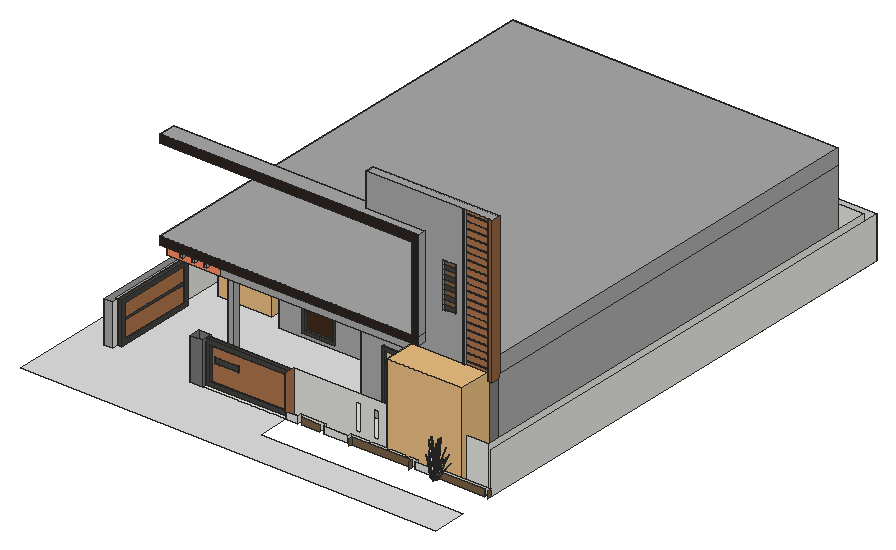
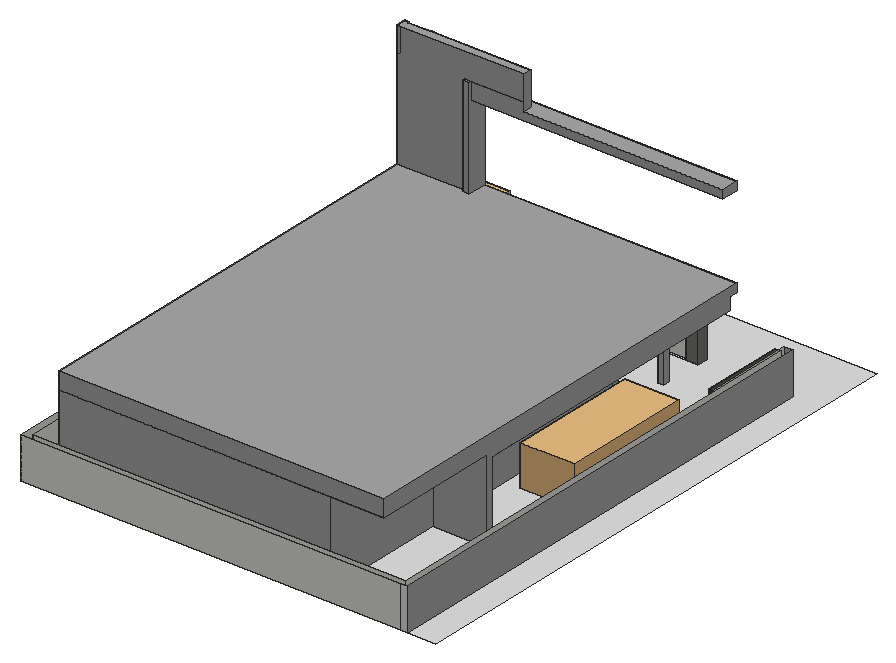
# SketchUp Ruby script. Lengths in inches.
U = 1.inch
M = Sketchup.active_model
def pt(a) = Geom::Point3d.new(a.map { |v| v * U })
def face(e, loops, mat)
  f = e.add_face(loops[0].map { |a| pt(a) })
  loops[1..].each { |l| e.add_face(l.map { |a| pt(a) }).erase! }
  f.material = f.back_material = mat if mat
  f
end
# faces: each face lists its corners as indices into pts; further lists are holes
def faces(e, pts, list, mat = nil) = list.each { |f| face(e, (f[0].is_a?(Array) ? f : [f]).map { |l| l.map { |i| pts[i] } }, mat) }
# xy, xz, yz: faces in a plane at the given z, y or x. An outline is a flat list of corners, or four numbers for a rectangle; further outlines are holes
def ring(l) = l.size == 4 ? [[l[0], l[1]], [l[2], l[1]], [l[2], l[3]], [l[0], l[3]]] : l.each_slice(2).to_a
def flat(e, list, mat, &to3) = list.each { |f| face(e, (f[0].is_a?(Array) ? f : [f]).map { |l| ring(l).map { |u, v| to3.(u, v) } }, mat) }
def xy(e, z, list, mat = nil) = flat(e, list, mat) { |x, y| [x, y, z] }
def xz(e, y, list, mat = nil) = flat(e, list, mat) { |x, z| [x, y, z] }
def yz(e, x, list, mat = nil) = flat(e, list, mat) { |y, z| [x, y, z] }
def lines(e, pts, list) = list.each { |a, b| e.add_line(pt(pts[a]), pt(pts[b])) }
# prism: a flat outline (further loops are holes) pulled along v
def prism(e, loops, v, mat = nil)
  f = face(e, loops, mat); d = Geom::Vector3d.new(v.map { |x| x * U })
  f.pushpull(f.normal.samedirection?(d) ? d.length : -d.length)
end
def box(e, o, s, mat = nil) = prism(e, [[o, [o[0] + s[0], o[1], o[2]], [o[0] + s[0], o[1] + s[1], o[2]], [o[0], o[1] + s[1], o[2]]]], [0, 0, s[2]], mat)
def at(x, y, z, deg = 0) = Geom::Transformation.translation(pt([x, y, z])) * Geom::Transformation.rotation(ORIGIN, Z_AXIS, deg.degrees)
def axes(o, x, y, z) = Geom::Transformation.new([*x, 0, *y, 0, *z, 0, *pt(o).to_a, 1])
def part(name) = M.definitions.add(name)
# library, detail: a bought-in or finely detailed component or shape, given as its bounding box
def library(name, o, s) = part(name).tap { |d| box(d.entities, o, s) }
def detail(e, o, s) = box(e.add_group.entities, o, s)
def put(e, d, t, mat = nil) = e.add_instance(d, t).tap { |i| i.material = mat if mat }
def group(e, t, mat = nil) = e.add_group.tap { |g| g.transformation = t; g.material = mat if mat }.entities
root = M.entities
M.materials.add("B03_Apricot_Glow").color = [255, 140, 101]
M.materials.add("Glass_Mirror_01").color = [226, 201, 168]
M.materials["Glass_Mirror_01"].alpha = 0.74
M.materials.add("Image").color = [118, 118, 115]
M.materials.add("M01_Silver_Fog").color = [224, 224, 224]
M.materials.add("M03_Pewter_Shine").color = [168, 168, 168]
M.materials.add("Plywood_01_1K").color = [125, 96, 64]
M.materials.add("Soil_03_1K").color = [122, 96, 67]
M.materials.add("Wood_Floor_12_1K").color = [45, 37, 32]
M.materials.add("Wood_Planks_01_1K").color = [69, 67, 63]
M.materials.add("Wood_Veneer_15_1K").color = [173, 116, 75]
M.materials.add("Wood_Veneer_15_1K1").color = [147, 99, 64]
M.materials.add("Wood_Veneer_15_1K2").color = [173, 116, 75]
M.materials.add("Wood_Veneer_15_1K3").color = [66, 44, 28]
c1 = part("blade")
p = [[2.15,0.21,22],[0,0.17,0],[0.09,0.45,0],[2.18,0.31,22],[2.29,0.31,22],[0.38,0.45,0],
  [2.48,0.24,33],[2.49,0.24,33],[2.48,0.22,33]]
faces(c1.entities,p,[[0,1,2,3],[4,5,2,3],[6,3,4,7],[8,0,3,6]])
c2 = part("blade with seeds\#1")
put(c2.entities,c1,at(0,0,0))
c3 = library("Baneira",[-21.22,-27.99,0],[51.24,48.13,67.625])
c4 = library("Car Sedan",[0,-0.48,0],[188.37,78.26,58.82])
xy(root,0,[[307.48,94.87,325.48,94.87,325.48,100.87,361.48,100.87,361.48,95.87,397.48,95.87,397.48,100.87,493.75,100.87,493.75,95.87,517.75,95.87,517.75,100.87,600,100.87,600,796.87,49.48,796.87,49.48,788.61,588.83,788.61,588.83,109.87,307.48,109.87],[169.48,94.87,187.48,109.87],[187.48,94.87,307.48,100.87],[187.48,100.87,307.48,109.87]])
xy(root,0,[[0,0,600.39,0,600.39,49.75,307.48,49.75,307.48,94.87,169.48,94.87,169.48,109.87,588.83,109.87,588.83,788.61,49.48,788.61,49.48,109.87,52.41,109.87,52.41,100.87,40.48,100.87,40.48,796.87,0,796.87]],"M01_Silver_Fog")
xz(root,94.87,[[307.48,0,325.48,10]])
xz(root,94.87,[[169.48,0,187.48,60]],"Image")
xz(root,95.87,[[361.48,0,397.48,10],[493.75,0,517.75,10]])
xz(root,95.87,[[330.48,0,356.48,10],[402.48,0,488.75,10],[522.75,0,595,10]],"Soil_03_1K")
xz(root,100.87,[[325.48,0,361.48,10],[397.48,0,493.75,0,493.75,10,482.46,10,482.46,9.35,475.45,9.35,475.45,10,456.47,10,456.47,9.35,449.46,9.35,449.46,10,430.48,10,430.48,9.35,423.47,9.35,423.47,10,404.48,10,404.48,9.35,397.48,9.35],[517.75,0,600,10]])
xz(root,100.87,[[40.48,0,52.41,60]],"M03_Pewter_Shine")
xz(root,109.87,[[49.48,0,52.41,60],[[307.48,0,588.83,60],[475.45,9.35,482.46,48],[449.46,9.35,456.47,48],[423.47,9.35,430.48,48],[397.48,9.35,404.48,48]]])
xz(root,109.87,[[169.48,0,187.48,60]],"Image")
xz(root,788.61,[[49.48,0,588.83,60]])
xz(root,796.87,[[40.48,0,49.48,60],[49.48,0,600,60]])
yz(root,40.48,[[100.87,0,796.87,60]],"M03_Pewter_Shine")
yz(root,49.48,[[109.87,0,788.61,60]])
yz(root,52.41,[[100.87,0,109.87,60]])
yz(root,169.48,[[94.87,0,109.87,60]],"Image")
yz(root,187.48,[[94.87,0,109.87,60]],"Image")
yz(root,307.48,[[94.87,0,109.87,60]],"Wood_Veneer_15_1K2")
yz(root,325.48,[[94.87,0,100.87,10]])
yz(root,361.48,[[95.87,0,100.87,10]])
yz(root,397.48,[[95.87,0,100.87,10]])
yz(root,402.48,[[90.87,0,95.87,10]],"Soil_03_1K")
yz(root,488.75,[[90.87,0,95.87,10]],"Soil_03_1K")
yz(root,493.75,[[95.87,0,100.87,10]])
yz(root,517.75,[[95.87,0,100.87,10]])
yz(root,522.75,[[90.87,0,95.87,10]],"Soil_03_1K")
yz(root,588.83,[[109.87,0,788.61,60]])
yz(root,595,[[94.87,0,95.87,10]],"Soil_03_1K")
yz(root,600,[[100.87,0,796.87,60]])
yz(root,600,[[94.87,0,100.87,10]],"Soil_03_1K")
put(root,c2,axes([527.79,90.97,3.51],[0.90375,0.03008,-0.71091],[-0.0607,1.26677,0.08579],[0.38287,0.13368,1.00565]))
put(root,c2,axes([526.65,87.39,1.69],[0.39398,-0.99907,1.36359],[0.84877,0.97875,0.53923],[-0.50305,0.4384,1.14314]))
put(root,c2,axes([519.51,91.2,1.1875],[0.34005,-0.60308,1.03545],[0.20441,0.87829,0.76078],[-0.26134,0.18792,0.22807]))
put(root,c2,axes([526.79,87.49,0.55],[0.73437,0.77871,-0.5621],[-0.66591,0.96736,-0.14753],[0.18319,0.31204,1.24074]))
put(root,c2,axes([524.38,91.8125,0.8],[0.82143,1.07538,0.27726],[-0.81279,1.07603,-0.32897],[-0.23327,0.03755,1.48641]))
put(root,c2,axes([527.44,90.9,0.52],[-0.85134,0.27158,-0.27926],[-0.24175,-1.0786,0.27926],[-0.09817,0.21744,1.25283]))
put(root,c2,axes([520.68,90.09,2.78],[-0.78697,0.17856,-0.31925],[-0.2078,-1.02074,0.41216],[-0.22552,0.27417,0.78863]))
put(root,c2,axes([528.33,91.49,2.78],[0.51441,0.78225,-0.31925],[-0.58738,0.7405,0.41216],[0.29843,0.11267,0.78863]))
put(root,c2,axes([526.08,88.26,1.1],[0.64866,1.16728,-0.26229],[-0.91655,0.77622,-0.45076],[-0.09308,0.288,1.43974]))
put(root,c2,axes([524.67,92.93,0.83],[0,1.44565,0],[-1.09198,0,-0.46523],[-0.24871,0,1.47583]))
put(root,c2,axes([520.02,90.85,1.03],[0.31962,0.07001,1.28914],[0.26756,1.02347,-0.27724],[-0.41311,0.23924,0.55117]))
put(root,c2,axes([529.81,91.86,1.03],[-0.15413,-0.36483,1.28914],[0.46474,-0.90077,-0.27724],[0.40213,0.2681,0.55117]))
put(root,c2,axes([521.03,92.38,0.61],[0.7978,0.33351,-0.03509],[-0.24541,1.02647,-0.15911],[-0.13049,0.15585,0.52479]))
put(root,c2,axes([528.4,90.54,0.83],[0.97904,0.72283,0],[-0.54599,1.20931,-0.46523],[-0.12435,0.27543,1.47583]))
put(root,c2,axes([527.81,91.2,0.51],[-0.48852,1.08202,-0.44759],[-0.87598,-0.64674,0],[-0.11126,0.24644,1.41987]))
put(root,c2,axes([521.31,89.75,3.1875],[-0.47225,0.98582,-0.64046],[-0.82754,-0.7006,0.07729],[-0.28197,0.35717,0.906]))
put(root,c2,axes([520.53,91.68,0.04],[0.12871,0.11199,1.5897],[0.2775,1.13173,-0.24285],[-0.25244,0.2734,0.27078]))
put(root,c2,axes([521.33,90.21,2.92],[0.23225,1.14083,-0.46065],[-0.87956,0.19957,-0.35681],[-0.25205,0.30642,0.88141]))
put(root,c2,axes([525.9375,89.625,0.55],[-0.16018,1.20264,-0.5621],[-0.98808,-0.25378,-0.14753],[-0.11973,0.3589,1.24074]))
put(root,c2,axes([526.58,92.43,2.92],[0.89213,-0.297,-0.46065],[0.15606,1.12475,-0.35681],[0.23962,0.32232,0.88141]))
put(root,c2,axes([528.85,93.81,0.04],[0.09761,-0.15508,1.5897],[0.90442,-0.26295,-0.24285],[0.19286,0.3437,0.27078]))
put(root,c2,axes([523.53,94.03,1.1875],[-0.06991,-0.73811,1.03545],[0.616,0.4682,0.76078],[-0.09241,0.36475,0.22807]))
put(root,c2,axes([526.48,93.26,2.78],[0.13963,1.00636,-0.31925],[-0.79822,0.26574,0.41216],[0.2144,0.28839,0.78863]))
put(root,c2,axes([528.4,95.08,1.1875],[-0.44281,-0.48182,1.03545],[0.70101,-0.19012,0.76078],[0.12552,0.34819,0.22807]))
put(root,c2,axes([522.68,92.14,2.92],[0.6472,0.83949,-0.46065],[-0.68369,0.73521,-0.35681],[-0.09847,0.42653,0.88141]))
put(root,c2,axes([524.54,93.49,0.04],[0.15398,-0.02932,1.5897],[0.80412,0.59108,-0.24285],[-0.04053,0.41985,0.27078]))
put(root,c2,axes([524.6,92.95,2.92],[0.88873,0.31321,-0.46065],[-0.30463,1.07385,-0.35681],[0.08149,0.43235,0.88141]))
put(root,c2,axes([524.19,93.61,2.78],[-0.27256,0.96081,-0.31925],[-0.79518,-0.28024,0.41216],[0.07291,0.38684,0.78863]))
put(root,c2,axes([522.48,91.76,3.1875],[-0.02352,1.1557,-0.64046],[-0.99061,-0.07762,0.07729],[-0.10454,0.48961,0.906]))
put(root,c2,axes([522.72,92.6875,1.03],[0.27202,-0.22572,1.28914],[0.7394,0.52014,-0.27724],[-0.17673,0.53408,0.55117]))
put(root,c2,axes([524.06,90.69,1.71],[-0.14134,-0.32863,1.5962],[0.98684,-0.11332,0.12492],[0.13095,0.71181,0.57049]))
put(root,c2,axes([526.68,94.24,1.03],[0.08021,-0.40179,1.28914],[0.81924,-0.25896,-0.27724],[0.15335,0.54576,0.55117]))
g1 = group(root,at(187.48,106.87,0))
xy(g1,0,[[0,-6,120,0]],"Wood_Planks_01_1K")
xy(g1,6,[[6,-6,114,-3]],"Wood_Planks_01_1K")
xy(g1,29.67,[[10.07,-3,45.08,-1.64]],"Wood_Planks_01_1K")
xy(g1,38.71,[[10.07,-3,45.08,-1.64]],"Wood_Planks_01_1K")
xy(g1,54,[[6,-6,114,-3]],"Wood_Planks_01_1K")
xy(g1,60,[[0,-6,120,0]],"Wood_Planks_01_1K")
xz(g1,-6,[[[0,0,120,60],[6,6,114,54]]],"Wood_Planks_01_1K")
xz(g1,-3,[[[6,6,114,54],[10.07,29.67,45.08,38.71]]],"Wood_Veneer_15_1K2")
xz(g1,-1.64,[[10.07,29.67,45.08,38.71]],"Wood_Planks_01_1K")
xz(g1,0,[[0,0,120,60]])
yz(g1,0,[[-6,0,0,60]],"Wood_Planks_01_1K")
yz(g1,6,[[-6,6,-3,54]],"Wood_Planks_01_1K")
yz(g1,10.07,[[-3,29.67,-1.64,38.71]],"Wood_Planks_01_1K")
yz(g1,45.08,[[-3,29.67,-1.64,38.71]],"Wood_Planks_01_1K")
yz(g1,114,[[-6,6,-3,54]],"Wood_Planks_01_1K")
yz(g1,120,[[-6,0,0,60]],"Wood_Planks_01_1K")
put(root,c3,axes([492.54,131.13,0],[2.1112,0,0],[0,1,0],[0,0,1.8357]))
g2 = group(root,at(52.41,109.87,0,90))
xy(g2,0,[[0,-6,120,0]],"Wood_Planks_01_1K")
xy(g2,6,[[6,-6,114,-3]],"Wood_Planks_01_1K")
xy(g2,54,[[6,-6,114,-3]],"Wood_Planks_01_1K")
xy(g2,60,[[0,-6,120,0]],"Wood_Planks_01_1K")
xz(g2,-6,[[[0,0,120,60],[6,6,114,54]]],"Wood_Planks_01_1K")
xz(g2,-3,[[6,28,114,32]],"Wood_Planks_01_1K")
xz(g2,-3,[[6,6,114,28],[6,32,114,54]],"Wood_Veneer_15_1K2")
xz(g2,0,[[0,0,120,60]])
yz(g2,0,[[-6,0,0,60]],"Wood_Planks_01_1K")
yz(g2,6,[[-6,6,-3,54]],"Wood_Planks_01_1K")
yz(g2,114,[[-6,6,-3,54]],"Wood_Planks_01_1K")
yz(g2,120,[[-6,0,0,60]],"Wood_Planks_01_1K")
put(root,c4,at(148.51,268.88,0,90))
g3 = group(root,at(129,160.87,120),"M03_Pewter_Shine")
xy(g3,-120,[[-36,418.1,50.06,427.58]])
xy(g3,-6,[[393.23,-13.66,393.23,-12.74,40.22,-12.74,40.22,0,435,0,435,-13.66,429,-13.66,429,-12,395.99,-12,395.99,-13.66],[-36,-12.74,-36,418.1,-24.58,418.1,-24.58,0,40.22,0,40.22,-12.74]])
xy(g3,0,[[-24.58,0,-24.58,418.1,50.06,418.1,50.06,427.58,-36,427.58,-36,612,435,612,435,0]])
xy(g3,0.01,[[-14.8125,-16,-10.09,-12.74],[2.7,-16,7.42,-12.74],[20.21,-16,24.93,-12.74]])
xy(g3,4.51,[[-14.8125,-16,-10.09,-12.74],[2.7,-16,7.42,-12.74],[20.21,-16,24.93,-12.74]])
xy(g3,12,[[-36,-24.39,337.47,-12.74]])
xy(g3,24,[[-36,-24.39,328.3125,-24.39,328.3125,3.12,337.47,3.12,337.47,0,435,0,435,612,-36,612]])
xy(g3,63.78,[[363.53,-12.74,381.62,-12]])
xy(g3,128.54,[[363.53,-12.74,381.62,-12]])
xy(g3,144,[[-36,-24.39,328.3125,0]],"Wood_Floor_12_1K")
xy(g3,156,[[-36,-24.39,337.47,-24.39,337.47,-12.74,252.48,-12.74,252.48,0,-36,0]])
xy(g3,168,[[328.3125,0,337.47,3.12]])
xy(g3,204,[[393.23,-13.66,395.99,-13.66,395.99,-12,429,-12,429,-13.66,435,-13.66,435,0,252.48,0,252.48,-12.74,393.23,-12.74]])
xz(g3,-24.39,[[-36,12,337.47,12,337.47,156,-36,156,-36,144,328.3125,144,328.3125,24,-36,24]],"Wood_Floor_12_1K")
xz(g3,-16,[[-14.8125,0.01,-10.09,4.51],[2.7,0.01,7.42,4.51],[20.21,0.01,24.93,4.51]])
xz(g3,-13.66,[[393.23,-6,395.99,204]])
xz(g3,-13.66,[[429,-6,435,204]],"Wood_Veneer_15_1K1")
xz(g3,-12.74,[[[40.22,-6,393.23,-6,393.23,204,252.48,204,252.48,156,337.47,156,337.47,12,39.74,12],[363.53,63.78,381.62,128.54]]])
xz(g3,-12.74,[[[-36,-6,40.22,-6,39.74,12,-36,12],[-14.8125,0.01,-10.09,4.51],[2.7,0.01,7.42,4.51],[20.21,0.01,24.93,4.51]]],"B03_Apricot_Glow")
xz(g3,-12,[[395.99,-1.84,429,-0.84],[395.99,8.2,429,9.2],[395.99,18.25,429,19.25],[395.99,28.29,429,29.29],[395.99,38.33,429,39.33],
  [395.99,48.37,429,49.37],[395.99,58.41,429,59.41],[395.99,68.46,429,69.46],[395.99,78.5,429,79.5],[395.99,88.54,429,89.54],
  [395.99,98.58,429,99.58],[395.99,108.625,429,109.625],[395.99,118.67,429,119.67],[395.99,128.71,429,129.71],[395.99,138.75,429,139.75],
  [395.99,148.79,429,149.79],[395.99,158.83,429,159.83],[395.99,168.875,429,169.875],[395.99,178.92,429,179.92],[395.99,188.96,429,189.96],
  [395.99,199,429,200]])
xz(g3,-12,[[363.53,70.26,381.62,76.74],[363.53,83.21,381.62,89.6875],[363.53,96.16,381.62,102.64],[363.53,109.11,381.62,115.59],[363.53,122.0625,381.62,128.54]],"Plywood_01_1K")
xz(g3,-12,[[363.53,63.78,381.62,70.26],[363.53,76.74,381.62,83.21],[363.53,89.6875,381.62,96.16],[363.53,102.64,381.62,109.11],[363.53,115.59,381.62,122.0625]],"Wood_Planks_01_1K")
xz(g3,-12,[[395.99,-6,429,-1.84],[395.99,-0.84,429,8.2],[395.99,9.2,429,18.25],[395.99,19.25,429,28.29],[395.99,29.29,429,38.33],
  [395.99,39.33,429,48.37],[395.99,49.37,429,58.41],[395.99,59.41,429,68.46],[395.99,69.46,429,78.5],[395.99,79.5,429,88.54],
  [395.99,89.54,429,98.58],[395.99,99.58,429,108.625],[395.99,109.625,429,118.67],[395.99,119.67,429,128.71],[395.99,129.71,429,138.75],
  [395.99,139.75,429,148.79],[395.99,149.79,429,158.83],[395.99,159.83,429,168.875],[395.99,169.875,429,178.92],[395.99,179.92,429,188.96],
  [395.99,189.96,429,199],[395.99,200,429,204]],"Wood_Veneer_15_1K")
xz(g3,0,[[-24.58,-6,435,0],[337.47,24,337.47,168,252.48,168,252.48,204,429,204,429,168,435,168,435,24],[-36,144,-36,156,252.48,156,252.48,168,328.3125,168,328.3125,144],[429,168,435,204]])
xz(g3,3.12,[[328.3125,24,337.47,168]])
xz(g3,418.1,[[-36,-120,50.06,-120,50.06,0,-24.58,0,-24.58,-6,-36,-6]])
xz(g3,427.58,[[-36,-120,50.06,0]])
xz(g3,612,[[-36,0,435,24]])
yz(g3,-36,[[418.1,-120,418.1,-6,-12.74,-6,-12.74,12,-24.39,12,-24.39,24,612,24,612,0,427.58,0,427.58,-120],[-24.39,144,0,156]])
yz(g3,-24.58,[[0,-6,418.1,0]])
yz(g3,-14.8125,[[-16,0.01,-12.74,4.51]])
yz(g3,-10.09,[[-16,0.01,-12.74,4.51]])
yz(g3,2.7,[[-16,0.01,-12.74,4.51]])
yz(g3,7.42,[[-16,0.01,-12.74,4.51]])
yz(g3,20.21,[[-16,0.01,-12.74,4.51]])
yz(g3,24.93,[[-16,0.01,-12.74,4.51]])
yz(g3,50.06,[[418.1,-120,427.58,0]])
yz(g3,252.48,[[-12.74,156,0,204]])
yz(g3,328.3125,[[-24.39,24,-24.39,144,0,144,0,168,3.12,168,3.12,24]])
yz(g3,337.47,[[-24.39,12,-12.74,24],[-24.39,24,-12.74,156],[0,24,3.12,168]])
yz(g3,363.53,[[-12.74,63.78,-12,70.26],[-12.74,70.26,-12,76.74],[-12.74,76.74,-12,83.21],[-12.74,83.21,-12,89.6875],[-12.74,89.6875,-12,96.16],
  [-12.74,96.16,-12,102.64],[-12.74,102.64,-12,109.11],[-12.74,109.11,-12,115.59],[-12.74,115.59,-12,122.0625],[-12.74,122.0625,-12,128.54]])
yz(g3,381.62,[[-12.74,63.78,-12,70.26],[-12.74,70.26,-12,76.74],[-12.74,76.74,-12,83.21],[-12.74,83.21,-12,89.6875],[-12.74,89.6875,-12,96.16],
  [-12.74,96.16,-12,102.64],[-12.74,102.64,-12,109.11],[-12.74,109.11,-12,115.59],[-12.74,115.59,-12,122.0625],[-12.74,122.0625,-12,128.54]])
yz(g3,393.23,[[-13.66,-6,-12.74,204]])
yz(g3,395.99,[[-13.66,-6,-12,204]])
yz(g3,429,[[-13.66,-6,-12,204]])
yz(g3,435,[[0,0,612,24]])
yz(g3,435,[[-13.66,-6,0,204]],"Wood_Veneer_15_1K1")
g4 = group(root,at(129,160.87,0),"M03_Pewter_Shine")
xy(g4,0,[[320.23,-2,435,-2,435,612,42,612,42,603,426,603,426,9,243,9,243,93,234,93,234,0,320.23,0],[243,9,426,93],[51,102,426,603]])
xy(g4,10,[[79,97.5,119,102]])
xy(g4,10,[[79,93,119,97.5]],"Wood_Planks_01_1K")
xy(g4,23.93,[[267.3,-3,315.71,0]])
xy(g4,27.93,[[271.3,-3,291.5,0],[295.5,-3,311.71,0]],"Wood_Planks_01_1K")
xy(g4,38.53,[[84.36,86.86,83.85,86.92,83.36,87.12,82.95,87.44,82.63,87.86,82.43,88.34,82.36,88.86,82.43,89.37,82.63,89.86,82.95,90.27,83.36,90.59,83.85,90.79,84.36,90.86,84.88,90.79,85.36,90.59,85.78,90.27,86.1,89.86,86.3,89.37,86.36,88.86,86.3,88.34,86.1,87.86,85.78,87.44,85.36,87.12,84.88,86.92]],"Wood_Veneer_15_1K3")
xy(g4,46,[[151,97.5,169,102],[173,97.5,191,102]])
xy(g4,46,[[151,93,169,97.5],[173,93,191,97.5]],"Wood_Planks_01_1K")
xy(g4,76.59,[[271.3,-3,291.5,0],[295.5,-3,311.71,0]])
xy(g4,80.59,[[271.3,-3,291.5,0],[295.5,-3,311.71,0]],"Wood_Planks_01_1K")
xy(g4,86,[[79,97.5,119,102],[151,97.5,169,102],[173,97.5,191,102]])
xy(g4,86,[[79,93,119,97.5],[151,93,169,97.5],[173,93,191,97.5]],"Wood_Planks_01_1K")
xy(g4,93.91,[[271.3,-3,291.5,0],[295.5,-3,311.71,0]])
xy(g4,97.91,[[267.3,-3,315.71,0]],"Wood_Planks_01_1K")
xy(g4,114,[[320.23,-2,435,0]])
xy(g4,120,[[41.58,0,50.58,10],[234,0,435,0,435,612,42,612,42,603,426,603,426,9,243,9,243,93,234,93],[41.58,93,42,102],[42,93,51,603],[51,93,426,102]])
xz(g4,-3,[[[267.3,23.93,315.71,97.91],[271.3,27.93,271.3,93.91,291.5,93.91,291.5,80.59,271.3,80.59,271.3,76.59,291.5,76.59,291.5,27.93],[295.5,27.93,295.5,76.59,311.71,76.59,311.71,80.59,295.5,80.59,295.5,93.91,311.71,93.91,311.71,27.93]]],"Wood_Planks_01_1K")
xz(g4,-2,[[320.23,0,435,114]],"Image")
xz(g4,0,[[41.58,0,50.58,120],[[234,0,320.23,0,320.23,114,435,114,435,120,234,120],[267.3,23.93,315.71,97.91]]])
xz(g4,0,[[271.3,27.93,291.5,76.59],[295.5,27.93,311.71,76.59],[271.3,80.59,291.5,93.91],[295.5,80.59,311.71,93.91]],"Glass_Mirror_01")
xz(g4,9,[[[243,0,426,120],[296,40,314,80]]])
xz(g4,10,[[41.58,0,50.58,120]])
xz(g4,89.09,[[84.36,38.02,84.88,38.09,85.36,38.29,85.78,38.61,86.1,39.02,86.3,39.5,86.36,40.02,86.3,40.54,86.1,41.02,85.78,41.43,85.36,41.75,84.88,41.95,84.36,42.02,83.85,41.95,83.36,41.75,82.95,41.43,82.63,41.02,82.43,40.54,82.36,40.02,82.43,39.5,82.63,39.02,82.95,38.61,83.36,38.29,83.85,38.09]],"Wood_Veneer_15_1K3")
xz(g4,93,[[41.58,0,42,120,41.58,120],[[41.58,0,234,0,234,120,42,120],[75,6,123,90],[147,42,195,90]],[234,0,243,120],[243,0,426,120]])
xz(g4,93,[[[75,6,123,90],[79,10,119,86]],[[147,42,195,90],[151,46,169,86],[173,46,191,86]]],"Wood_Planks_01_1K")
xz(g4,97.5,[[151,46,169,86],[173,46,191,86]],"Glass_Mirror_01")
xz(g4,97.5,[[[79,10,119,86],[84.36,52.44,84.88,52.51,85.36,52.71,85.78,53.03,86.1,53.44,86.3,53.93,86.36,54.44,86.3,54.96,86.1,55.44,85.78,55.86,85.36,56.18,84.88,56.375,84.36,56.44,83.85,56.375,83.36,56.18,82.95,55.86,82.63,55.44,82.43,54.96,82.36,54.44,82.43,53.93,82.63,53.44,82.95,53.03,83.36,52.71,83.85,52.51],[84.36,38.02,84.88,38.09,85.36,38.29,85.78,38.61,86.1,39.02,86.3,39.5,86.36,40.02,86.3,40.54,86.1,41.02,85.78,41.43,85.36,41.75,84.88,41.95,84.36,42.02,83.85,41.95,83.36,41.75,82.95,41.43,82.63,41.02,82.43,40.54,82.36,40.02,82.43,39.5,82.63,39.02,82.95,38.61,83.36,38.29,83.85,38.09]],[84.36,38.02,83.85,38.09,83.36,38.29,82.95,38.61,82.63,39.02,82.43,39.5,82.36,40.02,82.43,40.54,82.63,41.02,82.95,41.43,83.36,41.75,83.85,41.95,84.36,42.02,84.88,41.95,85.36,41.75,85.78,41.43,86.1,41.02,86.3,40.54,86.36,40.02,86.3,39.5,86.1,39.02,85.78,38.61,85.36,38.29,84.88,38.09],[84.36,52.44,83.85,52.51,83.36,52.71,82.95,53.03,82.63,53.44,82.43,53.93,82.36,54.44,82.43,54.96,82.63,55.44,82.95,55.86,83.36,56.18,83.85,56.375,84.36,56.44,84.88,56.375,85.36,56.18,85.78,55.86,86.1,55.44,86.3,54.96,86.36,54.44,86.3,53.93,86.1,53.44,85.78,53.03,85.36,52.71,84.88,52.51]],"Wood_Veneer_15_1K3")
xz(g4,102,[[41.58,0,42,120],[[51,0,426,120],[79,10,119,86],[151,46,169,86],[173,46,191,86]]])
xz(g4,603,[[51,0,396,120],[396,0,426,120]])
xz(g4,612,[[42,0,435,120]])
yz(g4,41.58,[[0,0,10,120],[93,0,102,120]])
yz(g4,42,[[102,0,612,120]])
yz(g4,50.58,[[0,0,10,120]])
yz(g4,51,[[102,0,603,120]])
yz(g4,79,[[97.5,10,102,86]])
yz(g4,79,[[93,10,97.5,86]],"Wood_Planks_01_1K")
yz(g4,119,[[97.5,10,102,86]])
yz(g4,119,[[93,10,97.5,86]],"Wood_Planks_01_1K")
yz(g4,151,[[97.5,46,102,86]])
yz(g4,151,[[93,46,97.5,86]],"Wood_Planks_01_1K")
yz(g4,169,[[97.5,46,102,86]])
yz(g4,169,[[93,46,97.5,86]],"Wood_Planks_01_1K")
yz(g4,173,[[97.5,46,102,86]])
yz(g4,173,[[93,46,97.5,86]],"Wood_Planks_01_1K")
yz(g4,191,[[97.5,46,102,86]])
yz(g4,191,[[93,46,97.5,86]],"Wood_Planks_01_1K")
yz(g4,234,[[0,0,93,120]])
yz(g4,243,[[9,0,93,120]])
yz(g4,267.3,[[-3,23.93,0,97.91]],"Wood_Planks_01_1K")
yz(g4,271.3,[[-3,76.59,0,80.59]])
yz(g4,271.3,[[-3,27.93,0,76.59],[-3,80.59,0,93.91]],"Wood_Planks_01_1K")
yz(g4,291.5,[[-3,27.93,0,76.59],[-3,80.59,0,93.91]],"Wood_Planks_01_1K")
yz(g4,295.5,[[-3,27.93,0,76.59],[-3,80.59,0,93.91]],"Wood_Planks_01_1K")
yz(g4,311.71,[[-3,76.59,0,80.59]])
yz(g4,311.71,[[-3,27.93,0,76.59],[-3,80.59,0,93.91]],"Wood_Planks_01_1K")
yz(g4,315.71,[[-3,23.93,0,97.91]],"Wood_Planks_01_1K")
yz(g4,320.23,[[-2,0,0,114]])
yz(g4,426,[[9,0,93,120],[93,0,102,120],[102,0,603,120]])
yz(g4,435,[[-2,0,612,0,612,120,0,120,0,114,-2,114]])
p = [[83.85,97.5,38.09],[84.36,97.5,38.02],[84.36,89.09,38.02],[83.85,89.09,38.09],[84.88,97.5,38.09],[84.88,89.09,38.09],
  [83.36,97.5,38.29],[83.36,89.09,38.29],[85.36,97.5,38.29],[85.36,89.09,38.29],[82.95,97.5,38.61],[82.95,89.09,38.61],
  [82.95,90.27,38.61],[85.78,97.5,38.61],[85.78,90.27,38.61],[85.78,89.09,38.61],[83.85,86.92,56.375],[83.36,87.12,56.18],
  [83.36,87.12,38.53],[83.85,86.92,38.53],[84.36,86.86,56.44],[84.36,86.86,38.53],[84.88,86.92,56.375],[84.88,86.92,38.53],
  [85.36,87.12,56.18],[85.36,87.12,38.53],[82.95,87.44,55.86],[82.95,87.44,38.53],[85.78,87.44,55.86],[85.78,87.44,38.53],
  [82.63,87.86,55.44],[82.63,87.86,38.53],[86.1,87.86,55.44],[86.1,87.86,38.53],[82.43,88.34,54.96],[82.43,88.34,38.53],
  [86.3,88.34,54.96],[86.3,88.34,38.53],[82.36,88.86,54.44],[82.36,88.86,38.53],[86.36,88.86,54.44],[86.36,88.86,38.53],
  [82.43,89.37,53.93],[82.43,89.37,40.54],[82.43,89.37,39.5],[82.43,89.37,38.53],[86.3,89.37,53.93],[86.3,89.37,38.53],
  [86.3,89.37,39.5],[86.3,89.37,40.54],[82.63,89.86,53.44],[82.63,89.86,41.02],[82.63,89.86,39.02],[82.63,89.86,38.53],
  [86.1,89.86,53.44],[86.1,89.86,38.53],[86.1,89.86,39.02],[86.1,89.86,41.02],[82.95,90.27,53.03],[82.95,90.27,41.43],
  [82.95,90.27,38.53],[85.78,90.27,53.03],[85.78,90.27,38.53],[85.78,90.27,41.43],[83.36,90.59,52.71],[83.36,90.59,41.75],
  [83.36,90.59,38.53],[85.36,90.59,52.71],[85.36,90.59,38.53],[85.36,90.59,41.75],[83.85,90.79,52.51],[83.85,90.79,41.95],
  [83.85,90.79,38.53],[84.88,90.79,52.51],[84.88,90.79,38.53],[84.88,90.79,41.95],[84.36,90.86,52.44],[84.36,90.86,42.02],
  [84.36,90.86,40.02],[84.36,90.86,38.53],[82.63,97.5,39.02],[82.63,89.09,39.02],[86.1,97.5,39.02],[86.1,89.09,39.02],
  [82.43,97.5,39.5],[82.43,89.09,39.5],[86.3,97.5,39.5],[86.3,89.09,39.5],[82.36,97.5,40.02],[82.36,89.09,40.02],
  [86.36,97.5,40.02],[86.36,89.09,40.02],[82.43,97.5,40.54],[82.43,89.09,40.54],[86.3,97.5,40.54],[86.3,89.09,40.54],
  [82.63,97.5,41.02],[82.63,89.09,41.02],[86.1,97.5,41.02],[86.1,89.09,41.02],[82.95,97.5,41.43],[82.95,89.09,41.43],
  [85.78,97.5,41.43],[85.78,89.09,41.43],[83.36,97.5,41.75],[83.36,89.09,41.75],[85.36,97.5,41.75],[85.36,89.09,41.75],
  [83.85,97.5,41.95],[83.85,89.09,41.95],[84.88,97.5,41.95],[84.88,89.09,41.95],[84.36,97.5,42.02],[84.36,89.09,42.02],
  [83.85,97.5,52.51],[84.36,97.5,52.44],[84.88,97.5,52.51],[83.36,97.5,52.71],[85.36,97.5,52.71],[82.95,97.5,53.03],
  [85.78,97.5,53.03],[82.63,97.5,53.44],[86.1,97.5,53.44],[82.43,97.5,53.93],[86.3,97.5,53.93],[82.36,97.5,54.44],
  [86.36,97.5,54.44],[82.43,97.5,54.96],[86.3,97.5,54.96],[82.63,97.5,55.44],[86.1,97.5,55.44],[82.95,97.5,55.86],
  [85.78,97.5,55.86],[83.36,97.5,56.18],[85.36,97.5,56.18],[83.85,97.5,56.375],[84.88,97.5,56.375],[84.36,97.5,56.44],
  [292,9,80],[292,9,40],[274,9,80],[292,0,40],[274,0,40],[274,9,40],
  [292,0,80],[274,0,80],[314,0,80],[314,9,80],[296,0,40],[296,9,40],
  [314,0,40],[314,9,40],[84.51,97.5,54.16],[84.51,104.7,54.16],[84.51,89.14,54.16],[84.51,89.14,42.59],
  [84.36,97.5,40.02],[84.51,89.14,41.15],[84.51,89.14,40.02],[84.51,89.14,39.96],[84.36,89.09,40.02]]
faces(g4,p,[[0,1,2,3],[1,4,5,2],[6,0,3,7],[4,8,9,5],[10,6,7,11,12],[8,13,14,15,9],[16,17,18,19],[20,16,19,21],
  [22,20,21,23],[24,22,23,25],[17,26,27,18],[28,24,25,29],[26,30,31,27],[32,28,29,33],[30,34,35,31],[36,32,33,37],
  [34,38,39,35],[40,36,37,41],[38,42,43,44,45,39],[46,40,41,47,48,49],[42,50,51,52,53,45,44,43],[54,46,49,48,47,55,56,57],[50,58,59,12,60,53,52,51],[61,54,57,56,55,62,14,63],
  [58,64,65,66,60,12,59],[67,61,63,14,62,68,69],[64,70,71,72,66,65],[73,67,69,68,74,75],[70,76,77,78,79,72,71],[76,73,75,74,79,78,77],[80,10,12,11,81,52],[13,82,56,83,15,14],
  [84,80,52,81,85,44],[82,86,48,87,83,56],[88,84,44,85,89],[86,90,91,87,48],[92,88,89,93,43],[90,94,49,95,91],[96,92,43,93,97,51],[94,98,57,99,95,49],
  [100,96,51,97,101,59],[98,102,63,103,99,57],[104,100,59,101,105,65],[102,106,69,107,103,63],[108,104,65,105,109,71],[106,110,75,111,107,69],[112,108,71,109,113,77],[110,112,77,113,111,75],
  [114,115,76,70],[115,116,73,76],[117,114,70,64],[116,118,67,73],[119,117,64,58],[118,120,61,67],[121,119,58,50],[120,122,54,61],
  [123,121,50,42],[122,124,46,54],[125,123,42,38],[124,126,40,46],[127,125,38,34],[126,128,36,40],[129,127,34,30],[128,130,32,36],
  [131,129,30,26],[130,132,28,32],[133,131,26,17],[132,134,24,28],[135,133,17,16],[134,136,22,24],[137,135,16,20],[136,137,20,22]],"Wood_Veneer_15_1K3")
lines(g4,p,[[138,139],[138,140],[141,139],[142,143],[144,138],[145,140],[146,147],[148,149],[150,151],[152,153],[154,152],[154,155],
  [156,78],[157,158],[158,159],[78,160]])
